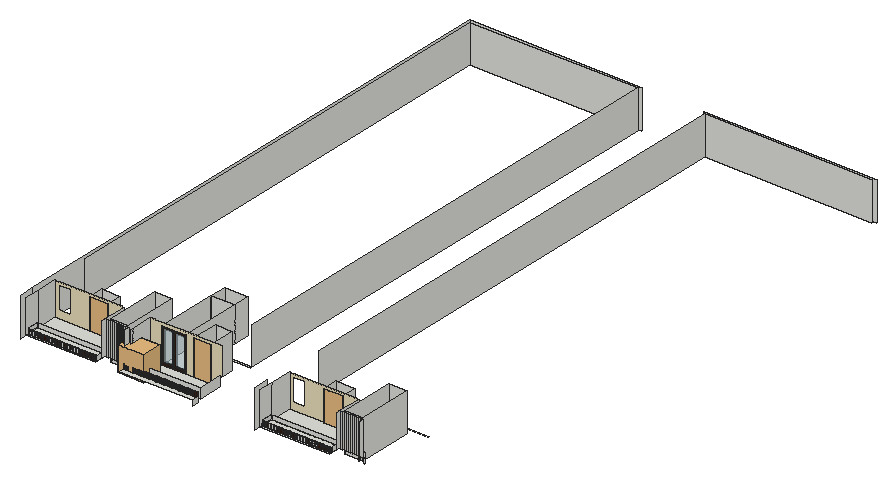
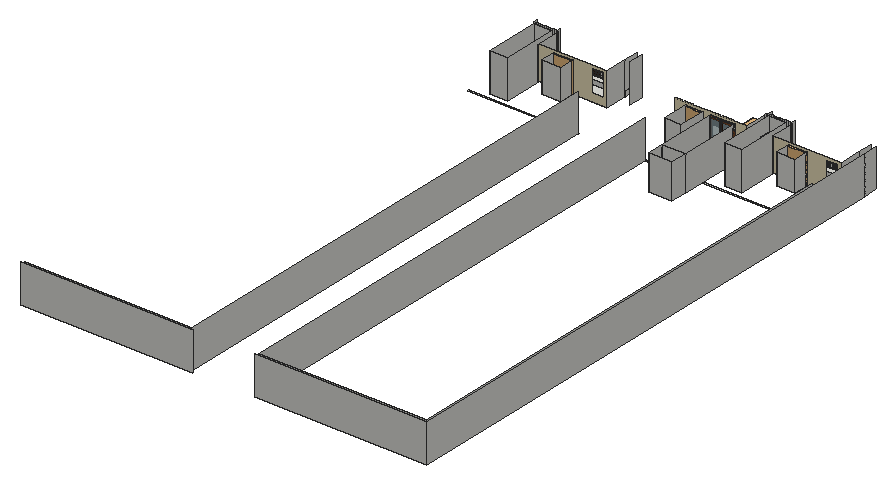
# SketchUp Ruby script. Lengths in inches.
U = 1.inch
M = Sketchup.active_model
def pt(a) = Geom::Point3d.new(a.map { |v| v * U })
def face(e, loops, mat)
  f = e.add_face(loops[0].map { |a| pt(a) })
  loops[1..].each { |l| e.add_face(l.map { |a| pt(a) }).erase! }
  f.material = f.back_material = mat if mat
  f
end
# faces: each face lists its corners as indices into pts; further lists are holes
def faces(e, pts, list, mat = nil) = list.each { |f| face(e, (f[0].is_a?(Array) ? f : [f]).map { |l| l.map { |i| pts[i] } }, mat) }
# xy, xz, yz: faces in a plane at the given z, y or x. An outline is a flat list of corners, or four numbers for a rectangle; further outlines are holes
def ring(l) = l.size == 4 ? [[l[0], l[1]], [l[2], l[1]], [l[2], l[3]], [l[0], l[3]]] : l.each_slice(2).to_a
def flat(e, list, mat, &to3) = list.each { |f| face(e, (f[0].is_a?(Array) ? f : [f]).map { |l| ring(l).map { |u, v| to3.(u, v) } }, mat) }
def xy(e, z, list, mat = nil) = flat(e, list, mat) { |x, y| [x, y, z] }
def xz(e, y, list, mat = nil) = flat(e, list, mat) { |x, z| [x, y, z] }
def yz(e, x, list, mat = nil) = flat(e, list, mat) { |y, z| [x, y, z] }
def lines(e, pts, list) = list.each { |a, b| e.add_line(pt(pts[a]), pt(pts[b])) }
# prism: a flat outline (further loops are holes) pulled along v
def prism(e, loops, v, mat = nil)
  f = face(e, loops, mat); d = Geom::Vector3d.new(v.map { |x| x * U })
  f.pushpull(f.normal.samedirection?(d) ? d.length : -d.length)
end
def box(e, o, s, mat = nil) = prism(e, [[o, [o[0] + s[0], o[1], o[2]], [o[0] + s[0], o[1] + s[1], o[2]], [o[0], o[1] + s[1], o[2]]]], [0, 0, s[2]], mat)
def at(x, y, z, deg = 0) = Geom::Transformation.translation(pt([x, y, z])) * Geom::Transformation.rotation(ORIGIN, Z_AXIS, deg.degrees)
def axes(o, x, y, z) = Geom::Transformation.new([*x, 0, *y, 0, *z, 0, *pt(o).to_a, 1])
def part(name) = M.definitions.add(name)
# library, detail: a bought-in or finely detailed component or shape, given as its bounding box
def library(name, o, s) = part(name).tap { |d| box(d.entities, o, s) }
def detail(e, o, s) = box(e.add_group.entities, o, s)
def put(e, d, t, mat = nil) = e.add_instance(d, t).tap { |i| i.material = mat if mat }
def group(e, t, mat = nil) = e.add_group.tap { |g| g.transformation = t; g.material = mat if mat }.entities
root = M.entities
M.materials.add("[Color D01]").color = [237, 225, 189]
M.materials.add("[Translucent Glass Safety]").color = [204, 235, 244]
M.materials["[Translucent Glass Safety]"].alpha = 0.5
M.materials.add("[Wood Veneer 01]").color = [51, 28, 15]
M.materials.add("[Wood Veneer 01]1").color = [120, 70, 37]
c1 = library("元件\#5",[-4.39,0,0],[5.37,35.83,90.55])
c2 = library("Round Planter with Plant",[-35.48,-39.77,0],[80.62,63.55,77.875])
c3 = part("Component\#1")
xy(c3.entities,0,[[0,0,6,48]],"[Wood Veneer 01]1")
xy(c3.entities,4,[[0,4,1.8125,44],[1.8125,4,6,44]])
xy(c3.entities,80,[[0,4,1.8125,44],[1.8125,4,6,44]])
xy(c3.entities,84,[[0,0,6,48]],"[Wood Veneer 01]1")
xz(c3.entities,0,[[0,0,6,84]],"[Wood Veneer 01]1")
xz(c3.entities,4,[[0,4,1.8125,80],[1.8125,4,6,80]])
xz(c3.entities,44,[[0,4,1.8125,80],[1.8125,4,6,80]])
xz(c3.entities,48,[[0,0,6,84]],"[Wood Veneer 01]1")
yz(c3.entities,0,[[[0,0,48,84],[4,4,44,80]]],"[Wood Veneer 01]1")
yz(c3.entities,1.8125,[[4,4,44,80]],"[Translucent Glass Safety]")
yz(c3.entities,6,[[[0,0,48,84],[4,4,44,80]]],"[Wood Veneer 01]")
c4 = part("Group\#3")
put(c4.entities,c3,at(0,0,0),"[Wood Veneer 01]")
g1 = group(c4.entities,at(0,48,0),"[Wood Veneer 01]")
xy(g1,0,[[0,0,6,48]],"[Wood Veneer 01]1")
xy(g1,4,[[0,4,1.8125,44],[1.8125,4,6,44]])
xy(g1,80,[[0,4,1.8125,44],[1.8125,4,6,44]])
xy(g1,84,[[0,0,6,48]],"[Wood Veneer 01]1")
xz(g1,0,[[0,0,6,84]],"[Wood Veneer 01]1")
xz(g1,4,[[0,4,1.8125,80],[1.8125,4,6,80]])
xz(g1,44,[[0,4,1.8125,80],[1.8125,4,6,80]])
xz(g1,48,[[0,0,6,84]],"[Wood Veneer 01]1")
yz(g1,0,[[[0,0,48,84],[4,4,44,80]]],"[Wood Veneer 01]1")
yz(g1,1.8125,[[4,4,44,80]],"[Translucent Glass Safety]")
yz(g1,6,[[[0,0,48,84],[4,4,44,80]]],"[Wood Veneer 01]")
xy(root,386.6875,[[396.57,286.21,614.76,361.27],[435.49,361.27,509.74,483.79],[534.92,361.27,587.67,445.08],[90.36,483.79,435.49,488.08],[435.49,483.79,509.74,551.2],
  [509.74,483.79,614.76,488.08],[823.93,483.79,1169.05,488.08],[435.49,551.2,509.74,604.39]])
xy(root,402.5,[[100.18,255.92,309.49,293.45],[833.74,255.92,1043.05,293.45],[100.18,293.45,315.43,293.45,315.43,361.27,266.47,361.27,266.47,408.14,207.81,408.14,207.81,361.27,100.18,361.27],[833.74,293.45,1049,293.45,1049,361.27,1000.03,361.27,1000.03,408.14,941.37,408.14,941.37,361.27,833.74,361.27]])
xy(root,403.1875,[[100.18,246.64,318.81,246.64,318.81,286.21,315.68,286.21,315.68,253.61,100.18,253.61],[393.95,246.64,622,246.64,622,266.43,398.72,266.43,398.72,263.8,393.95,263.8],[833.74,246.64,1052.37,246.64,1052.37,286.21,1049.24,286.21,1049.24,253.61,833.74,253.61],[100.18,253.61,309.49,255.92],[833.74,253.61,1043.05,255.92]])
xz(root,253.61,[[103.79,403.1875,104.93,416.75],[108.54,403.1875,109.68,416.75],[113.29,403.1875,114.43,416.75],[118.04,403.1875,119.18,416.75],[122.79,403.1875,123.93,416.75],
  [127.54,403.1875,128.68,416.75],[132.29,403.1875,133.43,416.75],[137.04,403.1875,138.18,416.75],[141.79,403.1875,142.93,416.75],[146.54,403.1875,147.68,416.75],
  [151.29,403.1875,152.43,416.75],[156.04,403.1875,157.18,416.75],[160.79,403.1875,161.93,416.75],[165.54,403.1875,166.68,416.75],[170.29,403.1875,171.43,416.75],
  [175.04,403.1875,176.18,416.75],[179.79,403.1875,180.93,416.75],[184.54,403.1875,185.68,416.75],[189.29,403.1875,190.43,416.75],[194.04,403.1875,195.18,416.75],
  [198.79,403.1875,199.93,416.75],[203.54,403.1875,204.68,416.75],[208.29,403.1875,209.43,416.75],[213.04,403.1875,214.18,416.75],[217.79,403.1875,218.93,416.75],
  [222.54,403.1875,223.68,416.75],[227.29,403.1875,228.43,416.75],[232.04,403.1875,233.18,416.75],[236.79,403.1875,237.93,416.75],[241.54,403.1875,242.68,416.75],
  [246.29,403.1875,247.43,416.75],[251.04,403.1875,252.18,416.75],[255.79,403.1875,256.93,416.75],[260.54,403.1875,261.68,416.75],[265.29,403.1875,266.43,416.75],
  [270.04,403.1875,271.18,416.75],[274.79,403.1875,275.93,416.75],[279.54,403.1875,280.68,416.75],[284.29,403.1875,285.43,416.75],[289.04,403.1875,290.18,416.75],
  [293.79,403.1875,294.93,416.75],[298.54,403.1875,299.68,416.75],[303.29,403.1875,304.43,416.75],[308.04,403.1875,309.18,416.75],[312.79,403.1875,313.93,416.75],
  [837.35,403.1875,838.49,416.75],[842.1,403.1875,843.24,416.75],[846.85,403.1875,847.99,416.75],[851.6,403.1875,852.74,416.75],[856.35,403.1875,857.49,416.75],
  [861.1,403.1875,862.24,416.75],[865.85,403.1875,866.99,416.75],[870.6,403.1875,871.74,416.75],[875.35,403.1875,876.49,416.75],[880.1,403.1875,881.24,416.75],
  [884.85,403.1875,885.99,416.75],[889.6,403.1875,890.74,416.75],[894.35,403.1875,895.49,416.75],[899.1,403.1875,900.24,416.75],[903.85,403.1875,904.99,416.75],
  [908.6,403.1875,909.74,416.75],[913.35,403.1875,914.49,416.75],[918.1,403.1875,919.24,416.75],[922.85,403.1875,923.99,416.75],[927.6,403.1875,928.74,416.75],
  [932.35,403.1875,933.49,416.75],[937.1,403.1875,938.24,416.75],[941.85,403.1875,942.99,416.75],[946.6,403.1875,947.74,416.75],[951.35,403.1875,952.49,416.75],
  [956.1,403.1875,957.24,416.75],[960.85,403.1875,961.99,416.75],[965.6,403.1875,966.74,416.75],[970.35,403.1875,971.49,416.75],[975.1,403.1875,976.24,416.75],
  [979.85,403.1875,980.99,416.75],[984.6,403.1875,985.74,416.75],[989.35,403.1875,990.49,416.75],[994.1,403.1875,995.24,416.75],[998.85,403.1875,999.99,416.75],
  [1003.6,403.1875,1004.74,416.75],[1008.35,403.1875,1009.49,416.75],[1013.1,403.1875,1014.24,416.75],[1017.85,403.1875,1018.99,416.75],[1022.6,403.1875,1023.74,416.75],
  [1027.35,403.1875,1028.49,416.75],[1032.1,403.1875,1033.24,416.75],[1036.85,403.1875,1037.99,416.75],[1041.6,403.1875,1042.74,416.75],[1046.35,403.1875,1047.49,416.75]])
xz(root,253.61,[[100.18,403.1875,103.79,416.75],[104.93,403.1875,108.54,416.75],[109.68,403.1875,113.29,416.75],[114.43,403.1875,118.04,416.75],[119.18,403.1875,122.79,416.75],
  [123.93,403.1875,127.54,416.75],[128.68,403.1875,132.29,416.75],[133.43,403.1875,137.04,416.75],[138.18,403.1875,141.79,416.75],[142.93,403.1875,146.54,416.75],
  [147.68,403.1875,151.29,416.75],[152.43,403.1875,156.04,416.75],[157.18,403.1875,160.79,416.75],[161.93,403.1875,165.54,416.75],[166.68,403.1875,170.29,416.75],
  [171.43,403.1875,175.04,416.75],[176.18,403.1875,179.79,416.75],[180.93,403.1875,184.54,416.75],[185.68,403.1875,189.29,416.75],[190.43,403.1875,194.04,416.75],
  [195.18,403.1875,198.79,416.75],[199.93,403.1875,203.54,416.75],[204.68,403.1875,208.29,416.75],[209.43,403.1875,213.04,416.75],[214.18,403.1875,217.79,416.75],
  [218.93,403.1875,222.54,416.75],[223.68,403.1875,227.29,416.75],[228.43,403.1875,232.04,416.75],[233.18,403.1875,236.79,416.75],[237.93,403.1875,241.54,416.75],
  [242.68,403.1875,246.29,416.75],[247.43,403.1875,251.04,416.75],[252.18,403.1875,255.79,416.75],[256.93,403.1875,260.54,416.75],[261.68,403.1875,265.29,416.75],
  [266.43,403.1875,270.04,416.75],[271.18,403.1875,274.79,416.75],[275.93,403.1875,279.54,416.75],[280.68,403.1875,284.29,416.75],[285.43,403.1875,289.04,416.75],
  [290.18,403.1875,293.79,416.75],[294.93,403.1875,298.54,416.75],[299.68,403.1875,303.29,416.75],[304.43,403.1875,308.04,416.75],[309.18,403.1875,312.79,416.75],
  [313.93,403.1875,315.68,416.75],[315.68,403.1875,317.54,416.75],[833.74,403.1875,837.35,416.75],[838.49,403.1875,842.1,416.75],[843.24,403.1875,846.85,416.75],
  [847.99,403.1875,851.6,416.75],[852.74,403.1875,856.35,416.75],[857.49,403.1875,861.1,416.75],[862.24,403.1875,865.85,416.75],[866.99,403.1875,870.6,416.75],
  [871.74,403.1875,875.35,416.75],[876.49,403.1875,880.1,416.75],[881.24,403.1875,884.85,416.75],[885.99,403.1875,889.6,416.75],[890.74,403.1875,894.35,416.75],
  [895.49,403.1875,899.1,416.75],[900.24,403.1875,903.85,416.75],[904.99,403.1875,908.6,416.75],[909.74,403.1875,913.35,416.75],[914.49,403.1875,918.1,416.75],
  [919.24,403.1875,922.85,416.75],[923.99,403.1875,927.6,416.75],[928.74,403.1875,932.35,416.75],[933.49,403.1875,937.1,416.75],[938.24,403.1875,941.85,416.75],
  [942.99,403.1875,946.6,416.75],[947.74,403.1875,951.35,416.75],[952.49,403.1875,956.1,416.75],[957.24,403.1875,960.85,416.75],[961.99,403.1875,965.6,416.75],
  [966.74,403.1875,970.35,416.75],[971.49,403.1875,975.1,416.75],[976.24,403.1875,979.85,416.75],[980.99,403.1875,984.6,416.75],[985.74,403.1875,989.35,416.75],
  [990.49,403.1875,994.1,416.75],[995.24,403.1875,998.85,416.75],[999.99,403.1875,1003.6,416.75],[1004.74,403.1875,1008.35,416.75],[1009.49,403.1875,1013.1,416.75],
  [1014.24,403.1875,1017.85,416.75],[1018.99,403.1875,1022.6,416.75],[1023.74,403.1875,1027.35,416.75],[1028.49,403.1875,1032.1,416.75],[1033.24,403.1875,1036.85,416.75],
  [1037.99,403.1875,1041.6,416.75],[1042.74,403.1875,1046.35,416.75],[1047.49,403.1875,1049.24,416.75],[1049.24,403.1875,1051.1,416.75]],"[Wood Veneer 01]")
xz(root,255.92,[[100.18,402.5,309.49,403.1875],[833.74,402.5,1043.05,403.1875]])
xz(root,263.8,[[393.95,403.1875,398.72,416.75],[399.95,403.1875,404.72,416.75],[405.95,403.1875,410.72,416.75],[411.95,403.1875,416.72,416.75],[417.95,403.1875,422.72,416.75],
  [423.95,403.1875,428.72,416.75],[429.95,403.1875,434.72,416.75],[435.95,403.1875,440.72,416.75],[441.95,403.1875,446.72,416.75],[447.95,403.1875,452.72,416.75],
  [453.95,403.1875,458.72,416.75],[459.95,403.1875,464.72,416.75],[465.95,403.1875,470.72,416.75],[471.95,403.1875,476.72,416.75],[477.95,403.1875,482.72,416.75],
  [483.95,403.1875,488.72,416.75],[489.95,403.1875,494.72,416.75],[495.95,403.1875,500.72,416.75],[501.95,403.1875,506.72,416.75],[507.95,403.1875,512.72,416.75],
  [513.95,403.1875,518.72,416.75],[519.95,403.1875,524.72,416.75],[525.95,403.1875,530.72,416.75],[531.95,403.1875,536.72,416.75],[537.95,403.1875,542.72,416.75],
  [543.95,403.1875,548.72,416.75],[549.95,403.1875,554.72,416.75],[555.95,403.1875,560.72,416.75],[561.95,403.1875,566.72,416.75],[567.95,403.1875,572.72,416.75],
  [573.95,403.1875,578.72,416.75],[579.95,403.1875,584.72,416.75],[585.95,403.1875,590.72,416.75],[591.95,403.1875,596.72,416.75],[597.95,403.1875,602.72,416.75],
  [603.95,403.1875,608.72,416.75],[609.95,403.1875,614.72,416.75],[615.95,403.1875,620.72,416.75],[1127.51,403.1875,1132.28,416.75]],"[Wood Veneer 01]")
xz(root,266.43,[[398.72,403.1875,404.72,416.75],[404.72,403.1875,410.72,416.75],[410.72,403.1875,416.72,416.75],[416.72,403.1875,422.72,416.75],[422.72,403.1875,428.72,416.75],
  [428.72,403.1875,434.72,416.75],[434.72,403.1875,440.72,416.75],[440.72,403.1875,446.72,416.75],[446.72,403.1875,452.72,416.75],[452.72,403.1875,458.72,416.75],
  [458.72,403.1875,464.72,416.75],[464.72,403.1875,470.72,416.75],[470.72,403.1875,476.72,416.75],[476.72,403.1875,482.72,416.75],[482.72,403.1875,488.72,416.75],
  [488.72,403.1875,494.72,416.75],[494.72,403.1875,500.72,416.75],[500.72,403.1875,506.72,416.75],[506.72,403.1875,512.72,416.75],[512.72,403.1875,518.72,416.75],
  [518.72,403.1875,524.72,416.75],[524.72,403.1875,530.72,416.75],[530.72,403.1875,536.72,416.75],[536.72,403.1875,542.72,416.75],[542.72,403.1875,548.72,416.75],
  [548.72,403.1875,554.72,416.75],[554.72,403.1875,560.72,416.75],[560.72,403.1875,566.72,416.75],[566.72,403.1875,572.72,416.75],[572.72,403.1875,578.72,416.75],
  [578.72,403.1875,584.72,416.75],[584.72,403.1875,590.72,416.75],[590.72,403.1875,596.72,416.75],[596.72,403.1875,602.72,416.75],[602.72,403.1875,608.72,416.75],
  [608.72,403.1875,614.72,416.75],[614.72,403.1875,614.76,416.75],[614.76,403.1875,620.72,416.75],[620.72,403.1875,622,416.75]])
xz(root,286.21,[[393.95,386.6875,396.57,403.1875],[396.57,386.6875,614.76,416.75],[1127.51,386.6875,1130.14,403.1875],[315.68,403.1875,318.81,403.1875,318.81,505.3125,315.43,505.3125,315.43,409.375,315.68,409.375],[393.95,403.1875,396.57,416.75],
  [1049.24,403.1875,1052.37,403.1875,1052.37,505.3125,1049,505.3125,1049,409.375,1049.24,409.375],[1127.51,403.1875,1130.14,416.75]])
xz(root,293.45,[[328.03,386.6875,382.74,506.6875],[1061.59,386.6875,1116.3,506.6875],[100.18,402.5,100.18,416.75,315.43,416.75,315.43,409.375,309.49,409.375,309.49,402.5],[309.49,402.5,315.43,409.375],[833.74,402.5,833.74,416.75,1049,416.75,1049,409.375,1043.05,409.375,1043.05,402.5],
  [1043.05,402.5,1049,409.375]])
xz(root,361.27,[[396.57,386.6875,435.49,386.6875,435.49,495.625,509.74,495.625,509.74,386.6875,534.92,386.6875,534.92,495.6875,587.67,495.6875,587.67,386.6875,614.76,386.6875,614.76,418.9375,622,418.9375,622,505.3125,615.78,505.3125,615.78,504,609.07,504,609.07,505.3125,607.28,505.3125,607.28,504,600.57,504,600.57,505.3125,598.78,505.3125,598.78,504,592.07,504,592.07,505.3125,590.28,505.3125,590.28,504,583.57,504,583.57,505.3125,581.78,505.3125,581.78,504,575.07,504,575.07,505.3125,573.28,505.3125,573.28,504,566.57,504,566.57,505.3125,564.78,505.3125,564.78,504,558.07,504,558.07,505.3125,556.28,505.3125,556.28,504,549.57,504,549.57,505.3125,547.78,505.3125,547.78,504,541.07,504,541.07,505.3125,539.28,505.3125,539.28,504,532.57,504,532.57,505.3125,530.78,505.3125,530.78,504,524.07,504,524.07,505.3125,522.28,505.3125,522.28,504,515.57,504,515.57,505.3125,513.78,505.3125,513.78,504,507.07,504,507.07,505.3125,505.28,505.3125,505.28,504,498.57,504,498.57,505.3125,496.78,505.3125,496.78,504,490.07,504,490.07,505.3125,488.28,505.3125,488.28,504,481.57,504,481.57,505.3125,479.78,505.3125,479.78,504,473.07,504,473.07,505.3125,471.28,505.3125,471.28,504,464.57,504,464.57,505.3125,462.78,505.3125,462.78,504,456.07,504,456.07,505.3125,454.28,505.3125,454.28,504,447.57,504,447.57,505.3125,445.78,505.3125,445.78,504,439.07,504,439.07,505.3125,437.28,505.3125,437.28,504,430.57,504,430.57,505.3125,428.78,505.3125,428.78,504,422.07,504,422.07,505.3125,420.28,505.3125,420.28,504,413.57,504,413.57,505.3125,411.78,505.3125,411.78,504,405.07,504,405.07,505.3125,403.28,505.3125,403.28,504,396.57,504],[[100.18,402.5,207.81,402.5,207.81,497.42,266.47,497.42,266.47,402.5,315.43,402.5,315.43,503.875,309.94,503.875,309.94,505.3125,307.43,505.3125,307.43,503.875,301.94,503.875,301.94,505.3125,299.43,505.3125,299.43,503.875,293.94,503.875,293.94,505.3125,291.43,505.3125,291.43,503.875,285.94,503.875,285.94,505.3125,283.43,505.3125,283.43,503.875,277.94,503.875,277.94,505.3125,275.43,505.3125,275.43,503.875,269.94,503.875,269.94,505.3125,267.43,505.3125,267.43,503.875,261.94,503.875,261.94,505.3125,259.43,505.3125,259.43,503.875,253.94,503.875,253.94,505.3125,251.43,505.3125,251.43,504,245.94,504,245.94,505.3125,243.43,505.3125,243.43,504,237.94,504,237.94,505.3125,235.43,505.3125,235.43,504,229.94,504,229.94,505.3125,227.43,505.3125,227.43,504,221.94,504,221.94,505.3125,219.43,505.3125,219.43,504,213.94,504,213.94,505.3125,211.43,505.3125,211.43,504,205.94,504,205.94,505.3125,203.43,505.3125,203.43,504,197.94,504,197.94,505.3125,195.43,505.3125,195.43,504,189.94,504,189.94,505.3125,187.43,505.3125,187.43,504,181.94,504,181.94,505.3125,179.43,505.3125,179.43,504,173.94,504,173.94,505.3125,171.43,505.3125,171.43,504,165.94,504,165.94,505.3125,163.43,505.3125,163.43,504,157.94,504,157.94,505.3125,155.43,505.3125,155.43,504,149.94,504,149.94,505.3125,147.43,505.3125,147.43,504,141.94,504,141.94,505.3125,139.43,505.3125,139.43,504,133.94,504,133.94,505.3125,131.43,505.3125,131.43,504,125.94,504,125.94,505.3125,123.43,505.3125,123.43,504,117.94,504,117.94,505.3125,115.43,505.3125,115.43,504,109.94,504,109.94,505.3125,100.18,505.3125],[111.92,425.31,149.24,497.43]],[[833.74,402.5,941.37,402.5,941.37,497.42,1000.03,497.42,1000.03,402.5,1049,402.5,1049,503.875,1043.51,503.875,1043.51,505.3125,1041,505.3125,1041,503.875,1035.51,503.875,1035.51,505.3125,1033,505.3125,1033,503.875,1027.51,503.875,1027.51,505.3125,1025,505.3125,1025,503.875,1019.51,503.875,1019.51,505.3125,1017,505.3125,1017,503.875,1011.51,503.875,1011.51,505.3125,1009,505.3125,1009,503.875,1003.51,503.875,1003.51,505.3125,1001,505.3125,1001,503.875,995.51,503.875,995.51,505.3125,993,505.3125,993,503.875,987.51,503.875,987.51,505.3125,985,505.3125,985,504,979.51,504,979.51,505.3125,977,505.3125,977,504,971.51,504,971.51,505.3125,969,505.3125,969,504,963.51,504,963.51,505.3125,961,505.3125,961,504,955.51,504,955.51,505.3125,953,505.3125,953,504,947.51,504,947.51,505.3125,945,505.3125,945,504,939.51,504,939.51,505.3125,937,505.3125,937,504,931.51,504,931.51,505.3125,929,505.3125,929,504,923.51,504,923.51,505.3125,921,505.3125,921,504,915.51,504,915.51,505.3125,913,505.3125,913,504,907.51,504,907.51,505.3125,905,505.3125,905,504,899.51,504,899.51,505.3125,897,505.3125,897,504,891.51,504,891.51,505.3125,889,505.3125,889,504,883.51,504,883.51,505.3125,881,505.3125,881,504,875.51,504,875.51,505.3125,873,505.3125,873,504,867.51,504,867.51,505.3125,865,505.3125,865,504,859.51,504,859.51,505.3125,857,505.3125,857,504,851.51,504,851.51,505.3125,849,505.3125,849,504,843.51,504,843.51,505.3125,833.74,505.3125],[845.49,425.31,882.8,497.43]]],"[Color D01]")
xz(root,408.14,[[207.81,402.5,266.47,497.42],[941.37,402.5,1000.03,497.42]])
xz(root,445.08,[[534.92,386.6875,587.67,495.6875]])
xz(root,465.02,[[328.03,386.6875,382.74,506.6875],[1061.59,386.6875,1116.3,506.6875]])
xz(root,551.2,[[435.49,386.6875,509.74,495.625]])
xz(root,604.39,[[435.49,386.6875,509.74,495.625]])
xz(root,1996.66,[[90.36,386.6875,614.76,506.6875],[823.93,386.6875,1348.32,506.6875]])
xz(root,2003.89,[[83.125,386.6875,622,506.6875],[816.6875,386.6875,1355.5625,506.6875]])
yz(root,83.125,[[246.64,386.6875,293.46,506.6875],[293.46,386.6875,2003.89,506.6875]])
yz(root,90.36,[[488.08,386.6875,1996.66,506.6875]])
yz(root,100.18,[[255.92,402.5,293.45,403.1875],[293.45,402.5,293.46,403.1875],[293.46,402.5,361.27,505.3125],[246.64,403.1875,253.61,403.1875,253.61,416.75,253.3,416.75,253.3,418.9375,293.45,418.9375,293.45,403.1875,293.46,403.1875,293.46,505.3125,246.64,505.3125],[253.61,403.1875,293.45,416.75]])
yz(root,207.81,[[361.27,402.5,408.14,497.42]])
yz(root,266.47,[[361.27,402.5,408.14,497.42]])
yz(root,315.43,[[293.45,402.5,361.27,503.875]])
yz(root,315.68,[[253.61,403.1875,286.21,403.1875,286.21,409.375,293.45,409.375,293.45,416.75,253.61,416.75]])
yz(root,318.81,[[271.96,403.1875,286.21,506.6875]])
yz(root,324.81,[[282.52,403.1875,286.21,506.6875]])
yz(root,328.03,[[293.45,386.6875,465.02,506.6875]])
yz(root,330.81,[[282.52,403.1875,286.21,506.6875]])
yz(root,336.81,[[282.52,403.1875,286.21,506.6875]])
yz(root,342.81,[[282.52,403.1875,286.21,506.6875]])
yz(root,348.81,[[283.46,403.1875,286.21,506.6875]])
yz(root,354.81,[[283.46,403.1875,286.21,506.6875]])
yz(root,360.81,[[283.46,403.1875,286.21,506.6875]])
yz(root,366.81,[[283.46,403.1875,286.21,506.6875]])
yz(root,372.81,[[283.46,403.1875,286.21,506.6875]])
yz(root,378.81,[[283.46,403.1875,286.21,506.6875]])
yz(root,382.74,[[293.45,386.6875,465.02,506.6875]])
yz(root,384.81,[[283.46,403.1875,286.21,506.6875]])
yz(root,390.12,[[272.89,403.1875,286.21,506.6875]])
yz(root,393.95,[[263.8,403.1875,266.49,416.75]],"[Wood Veneer 01]")
yz(root,396.57,[[286.21,386.6875,293.45,504],[293.45,386.6875,361.27,504]])
yz(root,398.72,[[263.8,403.1875,266.43,416.75]])
yz(root,404.72,[[263.8,403.1875,266.43,416.75]])
yz(root,410.72,[[263.8,403.1875,266.43,416.75]])
yz(root,416.72,[[263.8,403.1875,266.43,416.75]])
yz(root,422.72,[[263.8,403.1875,266.43,416.75]])
yz(root,428.72,[[263.8,403.1875,266.43,416.75]])
yz(root,434.72,[[263.8,403.1875,266.43,416.75]])
yz(root,435.49,[[361.27,386.6875,551.2,495.625],[551.2,386.6875,604.39,495.625]])
yz(root,440.72,[[263.8,403.1875,266.43,416.75]])
yz(root,446.72,[[263.8,403.1875,266.43,416.75]])
yz(root,452.72,[[263.8,403.1875,266.43,416.75]])
yz(root,458.72,[[263.8,403.1875,266.43,416.75]])
yz(root,464.72,[[263.8,403.1875,266.43,416.75]])
yz(root,470.72,[[263.8,403.1875,266.43,416.75]])
yz(root,476.72,[[263.8,403.1875,266.43,416.75]])
yz(root,482.72,[[263.8,403.1875,266.43,416.75]])
yz(root,488.72,[[263.8,403.1875,266.43,416.75]])
yz(root,494.72,[[263.8,403.1875,266.43,416.75]])
yz(root,500.72,[[263.8,403.1875,266.43,416.75]])
yz(root,506.72,[[263.8,403.1875,266.43,416.75]])
yz(root,509.74,[[361.27,386.6875,551.2,495.625],[551.2,386.6875,604.39,495.625]])
yz(root,512.72,[[263.8,403.1875,266.43,416.75]])
yz(root,518.72,[[263.8,403.1875,266.43,416.75]])
yz(root,524.72,[[263.8,403.1875,266.43,416.75]])
yz(root,530.72,[[263.8,403.1875,266.43,416.75]])
yz(root,534.92,[[361.27,386.6875,445.08,495.6875]])
yz(root,536.72,[[263.8,403.1875,266.43,416.75]])
yz(root,542.72,[[263.8,403.1875,266.43,416.75]])
yz(root,548.72,[[263.8,403.1875,266.43,416.75]])
yz(root,554.72,[[263.8,403.1875,266.43,416.75]])
yz(root,560.72,[[263.8,403.1875,266.43,416.75]])
yz(root,566.72,[[263.8,403.1875,266.43,416.75]])
yz(root,572.72,[[263.8,403.1875,266.43,416.75]])
yz(root,578.72,[[263.8,403.1875,266.43,416.75]])
yz(root,584.72,[[263.8,403.1875,266.43,416.75]])
yz(root,587.67,[[361.27,386.6875,445.08,495.6875]])
yz(root,590.72,[[263.8,403.1875,266.43,416.75]])
yz(root,596.72,[[263.8,403.1875,266.43,416.75]])
yz(root,602.72,[[263.8,403.1875,266.43,416.75]])
yz(root,608.72,[[263.8,403.1875,266.43,416.75]])
yz(root,614.76,[[286.21,386.6875,361.27,416.75],[488.08,386.6875,1996.66,506.6875]])
yz(root,622,[[246.64,386.6875,266.43,403.1875]])
yz(root,816.6875,[[246.64,386.6875,293.46,506.6875]])
yz(root,823.93,[[488.08,386.6875,1996.66,506.6875]])
yz(root,833.74,[[255.92,402.5,293.45,403.1875],[293.45,402.5,293.46,403.1875],[293.46,402.5,361.27,505.3125],[246.64,403.1875,253.61,403.1875,253.61,416.75,253.3,416.75,253.3,418.9375,293.45,418.9375,293.45,403.1875,293.46,403.1875,293.46,505.3125,246.64,505.3125],[253.61,403.1875,293.45,416.75]])
yz(root,941.37,[[361.27,402.5,408.14,497.42]])
yz(root,1000.03,[[361.27,402.5,408.14,497.42]])
yz(root,1049,[[293.45,402.5,361.27,503.875]])
yz(root,1049.24,[[253.61,403.1875,286.21,403.1875,286.21,409.375,293.45,409.375,293.45,416.75,253.61,416.75]])
yz(root,1052.37,[[271.96,403.1875,286.21,506.6875]])
yz(root,1058.37,[[282.52,403.1875,286.21,506.6875]])
yz(root,1061.59,[[293.45,386.6875,465.02,506.6875]])
yz(root,1064.37,[[282.52,403.1875,286.21,506.6875]])
yz(root,1070.37,[[282.52,403.1875,286.21,506.6875]])
yz(root,1076.37,[[282.52,403.1875,286.21,506.6875]])
yz(root,1082.37,[[283.46,403.1875,286.21,506.6875]])
yz(root,1088.37,[[283.46,403.1875,286.21,506.6875]])
yz(root,1094.37,[[283.46,403.1875,286.21,506.6875]])
yz(root,1100.37,[[283.46,403.1875,286.21,506.6875]])
yz(root,1106.37,[[283.46,403.1875,286.21,506.6875]])
yz(root,1112.37,[[283.46,403.1875,286.21,506.6875]])
yz(root,1116.3,[[293.45,386.6875,465.02,506.6875]])
yz(root,1118.37,[[283.46,403.1875,286.21,506.6875]])
yz(root,1123.68,[[272.89,403.1875,286.21,506.6875]])
yz(root,1127.51,[[263.8,403.1875,266.49,416.75]],"[Wood Veneer 01]")
put(root,c1,axes([207.81,361.64,402.5],[0,-1,0],[1.63746,0,0],[0,0,1.04827]))
put(root,c2,at(409.81,303,386.6875))
put(root,c4,axes([435.49,367.27,386.6875],[0,-1,0],[0.77344,0,0],[0,0,1.29687]))
put(root,c1,axes([535.46,362.12,386.6875],[0,-0.89,0],[1.45734,0,0],[0,0,1.20374]))
put(root,c1,axes([941.37,361.64,402.5],[0,-1,0],[1.63746,0,0],[0,0,1.04827]))
